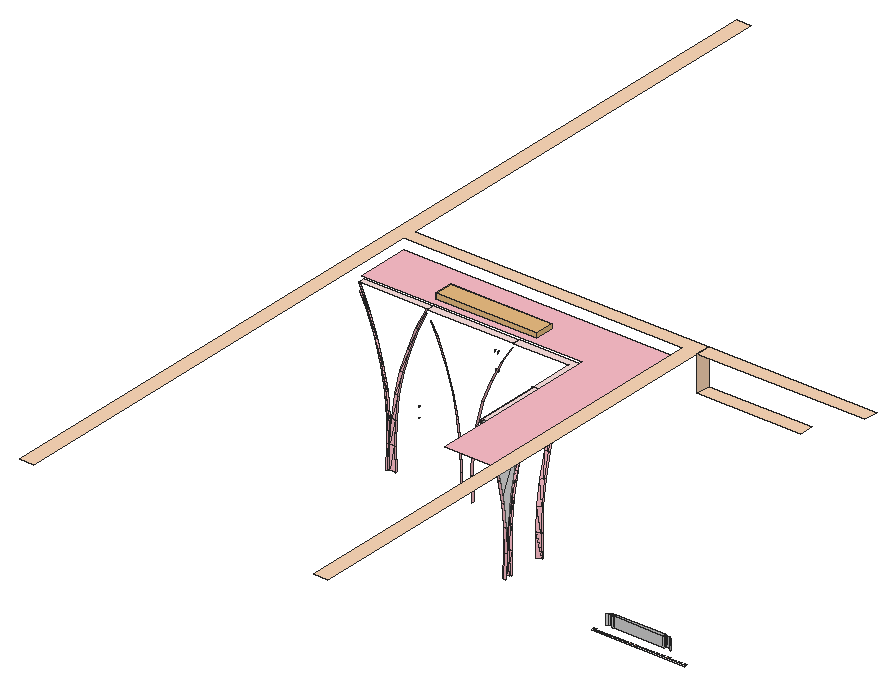
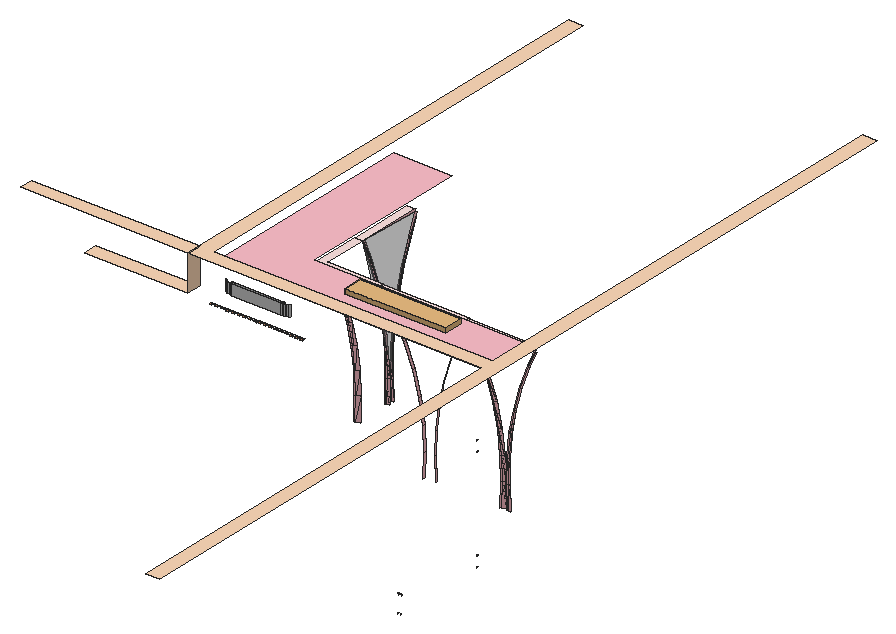
# SketchUp Ruby script. Lengths in inches.
U = 1.inch
M = Sketchup.active_model
def pt(a) = Geom::Point3d.new(a.map { |v| v * U })
def face(e, loops, mat)
  f = e.add_face(loops[0].map { |a| pt(a) })
  loops[1..].each { |l| e.add_face(l.map { |a| pt(a) }).erase! }
  f.material = f.back_material = mat if mat
  f
end
# faces: each face lists its corners as indices into pts; further lists are holes
def faces(e, pts, list, mat = nil) = list.each { |f| face(e, (f[0].is_a?(Array) ? f : [f]).map { |l| l.map { |i| pts[i] } }, mat) }
# xy, xz, yz: faces in a plane at the given z, y or x. An outline is a flat list of corners, or four numbers for a rectangle; further outlines are holes
def ring(l) = l.size == 4 ? [[l[0], l[1]], [l[2], l[1]], [l[2], l[3]], [l[0], l[3]]] : l.each_slice(2).to_a
def flat(e, list, mat, &to3) = list.each { |f| face(e, (f[0].is_a?(Array) ? f : [f]).map { |l| ring(l).map { |u, v| to3.(u, v) } }, mat) }
def xy(e, z, list, mat = nil) = flat(e, list, mat) { |x, y| [x, y, z] }
def xz(e, y, list, mat = nil) = flat(e, list, mat) { |x, z| [x, y, z] }
def yz(e, x, list, mat = nil) = flat(e, list, mat) { |y, z| [x, y, z] }
def lines(e, pts, list) = list.each { |a, b| e.add_line(pt(pts[a]), pt(pts[b])) }
# prism: a flat outline (further loops are holes) pulled along v
def prism(e, loops, v, mat = nil)
  f = face(e, loops, mat); d = Geom::Vector3d.new(v.map { |x| x * U })
  f.pushpull(f.normal.samedirection?(d) ? d.length : -d.length)
end
def box(e, o, s, mat = nil) = prism(e, [[o, [o[0] + s[0], o[1], o[2]], [o[0] + s[0], o[1] + s[1], o[2]], [o[0], o[1] + s[1], o[2]]]], [0, 0, s[2]], mat)
def at(x, y, z, deg = 0) = Geom::Transformation.translation(pt([x, y, z])) * Geom::Transformation.rotation(ORIGIN, Z_AXIS, deg.degrees)
def axes(o, x, y, z) = Geom::Transformation.new([*x, 0, *y, 0, *z, 0, *pt(o).to_a, 1])
def part(name) = M.definitions.add(name)
# library, detail: a bought-in or finely detailed component or shape, given as its bounding box
def library(name, o, s) = part(name).tap { |d| box(d.entities, o, s) }
def detail(e, o, s) = box(e.add_group.entities, o, s)
def put(e, d, t, mat = nil) = e.add_instance(d, t).tap { |i| i.material = mat if mat }
def group(e, t, mat = nil) = e.add_group.tap { |g| g.transformation = t; g.material = mat if mat }.entities
root = M.entities
M.materials.add("Material \#1").color = [140, 140, 140]
M.materials.add("[0006_Pink]").color = [255, 192, 203]
M.materials.add("[0007_MistyRose]").color = [255, 228, 225]
M.materials.add("[0010_Snow]").color = [255, 250, 250]
M.materials.add("[0027_PeachPuff]").color = [255, 218, 185]
M.materials.add("[Carrera Marble]").color = [207, 207, 207]
M.materials.add("[Translucent Glass Gray]").color = [128, 128, 128]
M.materials["[Translucent Glass Gray]"].alpha = 0.5
M.materials.add("[Wood Veneer 02]").color = [190, 128, 91]
c1 = library("wardrobe",[0.19,0,0],[43.3,8.22,2])
xy(root,47.11,[[363.16,355.99,363.12,356,363.12,356.03],[363.16,355.99,363.12,356.03,363.16,356.01],[363.16,355.99,363.16,356.01,363.2,356],[363.12,356,363.08,356.05,363.09,356.07],[363.12,356,363.09,356.07,363.12,356.03],
  [363.2,356,363.16,356.01,363.19,356.03],[363.2,356,363.19,356.03,363.23,356.05],[363.19,356.03,363.22,356.07,363.23,356.05],[363.08,356.05,363.06,356.12,363.07,356.13],[363.08,356.05,363.07,356.13,363.09,356.07],
  [363.23,356.05,363.22,356.07,363.26,356.12],[363.22,356.07,363.25,356.13,363.26,356.12],[363.06,356.12,363.04,356.2,363.06,356.2],[363.06,356.12,363.06,356.2,363.07,356.13],[363.26,356.12,363.25,356.13,363.27,356.2],
  [363.25,356.13,363.26,356.2,363.27,356.2],[363.04,356.2,363.04,356.29,363.06,356.28],[363.04,356.2,363.06,356.28,363.06,356.2],[363.26,356.2,363.26,356.28,363.27,356.29],[363.26,356.2,363.27,356.29,363.27,356.2],
  [363.06,356.28,363.04,356.29,363.07,356.36],[363.26,356.28,363.25,356.36,363.26,356.37],[363.26,356.28,363.26,356.37,363.27,356.29],[363.04,356.29,363.06,356.37,363.07,356.36],[363.07,356.36,363.06,356.37,363.09,356.42],
  [363.25,356.36,363.22,356.42,363.23,356.4375],[363.25,356.36,363.23,356.4375,363.26,356.37],[363.06,356.37,363.08,356.4375,363.09,356.42],[363.09,356.42,363.08,356.4375,363.12,356.46],[363.22,356.42,363.19,356.46,363.2,356.48],
  [363.22,356.42,363.2,356.48,363.23,356.4375],[363.08,356.4375,363.12,356.48,363.12,356.46],[363.12,356.46,363.12,356.48,363.16,356.47],[363.19,356.46,363.16,356.47,363.16,356.49],[363.19,356.46,363.16,356.49,363.2,356.48],
  [363.16,356.47,363.12,356.48,363.16,356.49]],"Material \#1")
xy(root,47.125,[[363.16,355.99,363.16,356.01,363.12,356],[363.16,355.99,363.19,356.03,363.16,356.01],[363.16,355.99,363.2,356,363.19,356.03],[363.12,356,363.12,356.03,363.08,356.05],[363.12,356,363.16,356.01,363.12,356.03],
  [363.2,356,363.22,356.07,363.19,356.03],[363.2,356,363.23,356.05,363.22,356.07],[363.12,356.03,363.09,356.07,363.08,356.05],[363.08,356.05,363.09,356.07,363.06,356.12],[363.23,356.05,363.25,356.13,363.22,356.07],
  [363.23,356.05,363.26,356.12,363.25,356.13],[363.09,356.07,363.07,356.13,363.06,356.12],[363.06,356.12,363.07,356.13,363.04,356.2],[363.26,356.12,363.26,356.2,363.25,356.13],[363.26,356.12,363.27,356.2,363.26,356.2],
  [363.07,356.13,363.06,356.2,363.04,356.2],[363.04,356.2,363.06,356.2,363.04,356.29],[363.06,356.2,363.06,356.28,363.04,356.29],[363.26,356.2,363.27,356.2,363.26,356.28],[363.27,356.2,363.27,356.29,363.26,356.28],
  [363.06,356.28,363.06,356.37,363.04,356.29],[363.06,356.28,363.07,356.36,363.06,356.37],[363.26,356.28,363.27,356.29,363.25,356.36],[363.27,356.29,363.26,356.37,363.25,356.36],[363.07,356.36,363.08,356.4375,363.06,356.37],
  [363.07,356.36,363.09,356.42,363.08,356.4375],[363.25,356.36,363.26,356.37,363.22,356.42],[363.26,356.37,363.23,356.4375,363.22,356.42],[363.09,356.42,363.12,356.48,363.08,356.4375],[363.09,356.42,363.12,356.46,363.12,356.48],
  [363.22,356.42,363.23,356.4375,363.19,356.46],[363.23,356.4375,363.2,356.48,363.19,356.46],[363.12,356.46,363.16,356.47,363.16,356.49],[363.12,356.46,363.16,356.49,363.12,356.48],[363.19,356.46,363.2,356.48,363.16,356.47],
  [363.16,356.47,363.2,356.48,363.16,356.49]],"Material \#1")
xy(root,50.26,[[502.06,274.78,521.41,275.36],[521.88,274.78,542,275.36]],"[0010_Snow]")
xy(root,50.26,[[502.06,275.36,503.17,276.11],[504.3,275.36,505.41,276.11],[506.54,275.36,507.65,276.11],[508.78,275.36,509.89,276.11],[511.02,275.36,512.13,276.11],
  [513.26,275.36,514.37,276.11],[515.5,275.36,516.61,276.11],[517.74,275.36,518.85,276.11],[519.98,275.36,521.09,276.11],[521.88,275.36,522.99,276.11],
  [524.26,275.36,525.37,276.11],[526.63,275.36,527.74,276.11],[529.01,275.36,530.12,276.11],[531.38,275.36,532.5,276.11],[533.76,275.36,534.87,276.11],
  [536.13,275.36,537.25,276.11],[538.51,275.36,539.62,276.11],[540.89,275.36,542,276.11]],"[Wood Veneer 02]")
xy(root,51.55,[[363.16,355.99,363.12,356,363.16,356.01],[363.16,355.99,363.16,356.01,363.19,356.03],[363.16,355.99,363.19,356.03,363.2,356],[363.12,356,363.08,356.05,363.12,356.03],[363.12,356,363.12,356.03,363.16,356.01],
  [363.2,356,363.19,356.03,363.22,356.07],[363.2,356,363.22,356.07,363.23,356.05],[363.12,356.03,363.08,356.05,363.09,356.07],[363.08,356.05,363.06,356.12,363.09,356.07],[363.23,356.05,363.22,356.07,363.25,356.13],
  [363.23,356.05,363.25,356.13,363.26,356.12],[363.09,356.07,363.06,356.12,363.07,356.13],[363.06,356.12,363.04,356.2,363.07,356.13],[363.26,356.12,363.25,356.13,363.26,356.2],[363.26,356.12,363.26,356.2,363.27,356.2],
  [363.07,356.13,363.04,356.2,363.06,356.2],[363.04,356.2,363.04,356.29,363.06,356.2],[363.06,356.2,363.04,356.29,363.06,356.28],[363.26,356.2,363.26,356.28,363.27,356.2],[363.27,356.2,363.26,356.28,363.27,356.29],
  [363.06,356.28,363.04,356.29,363.06,356.37],[363.06,356.28,363.06,356.37,363.07,356.36],[363.26,356.28,363.25,356.36,363.27,356.29],[363.27,356.29,363.25,356.36,363.26,356.37],[363.07,356.36,363.06,356.37,363.08,356.4375],
  [363.07,356.36,363.08,356.4375,363.09,356.42],[363.25,356.36,363.22,356.42,363.26,356.37],[363.26,356.37,363.22,356.42,363.23,356.4375],[363.09,356.42,363.08,356.4375,363.12,356.48],[363.09,356.42,363.12,356.48,363.12,356.46],
  [363.22,356.42,363.19,356.46,363.23,356.4375],[363.23,356.4375,363.19,356.46,363.2,356.48],[363.12,356.46,363.12,356.48,363.16,356.49],[363.12,356.46,363.16,356.49,363.16,356.47],[363.19,356.46,363.16,356.47,363.2,356.48],
  [363.16,356.47,363.16,356.49,363.2,356.48]],"Material \#1")
xy(root,51.57,[[363.16,355.99,363.12,356.03,363.12,356],[363.16,355.99,363.16,356.01,363.12,356.03],[363.16,355.99,363.2,356,363.16,356.01],[363.12,356,363.09,356.07,363.08,356.05],[363.12,356,363.12,356.03,363.09,356.07],
  [363.2,356,363.19,356.03,363.16,356.01],[363.2,356,363.23,356.05,363.19,356.03],[363.19,356.03,363.23,356.05,363.22,356.07],[363.08,356.05,363.07,356.13,363.06,356.12],[363.08,356.05,363.09,356.07,363.07,356.13],
  [363.23,356.05,363.26,356.12,363.22,356.07],[363.22,356.07,363.26,356.12,363.25,356.13],[363.06,356.12,363.06,356.2,363.04,356.2],[363.06,356.12,363.07,356.13,363.06,356.2],[363.26,356.12,363.27,356.2,363.25,356.13],
  [363.25,356.13,363.27,356.2,363.26,356.2],[363.04,356.2,363.06,356.2,363.06,356.28],[363.04,356.2,363.06,356.28,363.04,356.29],[363.26,356.2,363.27,356.2,363.27,356.29],[363.26,356.2,363.27,356.29,363.26,356.28],
  [363.06,356.28,363.07,356.36,363.04,356.29],[363.26,356.28,363.26,356.37,363.25,356.36],[363.26,356.28,363.27,356.29,363.26,356.37],[363.04,356.29,363.07,356.36,363.06,356.37],[363.07,356.36,363.09,356.42,363.06,356.37],
  [363.25,356.36,363.23,356.4375,363.22,356.42],[363.25,356.36,363.26,356.37,363.23,356.4375],[363.06,356.37,363.09,356.42,363.08,356.4375],[363.09,356.42,363.12,356.46,363.08,356.4375],[363.22,356.42,363.2,356.48,363.19,356.46],
  [363.22,356.42,363.23,356.4375,363.2,356.48],[363.08,356.4375,363.12,356.46,363.12,356.48],[363.12,356.46,363.16,356.47,363.12,356.48],[363.19,356.46,363.16,356.49,363.16,356.47],[363.19,356.46,363.2,356.48,363.16,356.49],
  [363.16,356.47,363.16,356.49,363.12,356.48]],"Material \#1")
xy(root,91.49,[[363.16,355.99,363.12,356,363.12,356.03],[363.16,355.99,363.12,356.03,363.16,356.01],[363.16,355.99,363.16,356.01,363.2,356],[363.12,356,363.08,356.05,363.09,356.07],[363.12,356,363.09,356.07,363.12,356.03],
  [363.2,356,363.16,356.01,363.19,356.03],[363.2,356,363.19,356.03,363.23,356.05],[363.19,356.03,363.22,356.07,363.23,356.05],[363.08,356.05,363.06,356.12,363.07,356.13],[363.08,356.05,363.07,356.13,363.09,356.07],
  [363.23,356.05,363.22,356.07,363.26,356.12],[363.22,356.07,363.25,356.13,363.26,356.12],[363.06,356.12,363.04,356.2,363.06,356.2],[363.06,356.12,363.06,356.2,363.07,356.13],[363.26,356.12,363.25,356.13,363.27,356.2],
  [363.25,356.13,363.26,356.2,363.27,356.2],[363.04,356.2,363.04,356.29,363.06,356.28],[363.04,356.2,363.06,356.28,363.06,356.2],[363.26,356.2,363.26,356.28,363.27,356.29],[363.26,356.2,363.27,356.29,363.27,356.2],
  [363.06,356.28,363.04,356.29,363.07,356.36],[363.26,356.28,363.25,356.36,363.26,356.37],[363.26,356.28,363.26,356.37,363.27,356.29],[363.04,356.29,363.06,356.37,363.07,356.36],[363.07,356.36,363.06,356.37,363.09,356.42],
  [363.25,356.36,363.22,356.42,363.23,356.4375],[363.25,356.36,363.23,356.4375,363.26,356.37],[363.06,356.37,363.08,356.4375,363.09,356.42],[363.09,356.42,363.08,356.4375,363.12,356.46],[363.22,356.42,363.19,356.46,363.2,356.48],
  [363.22,356.42,363.2,356.48,363.23,356.4375],[363.08,356.4375,363.12,356.48,363.12,356.46],[363.12,356.46,363.12,356.48,363.16,356.47],[363.19,356.46,363.16,356.47,363.16,356.49],[363.19,356.46,363.16,356.49,363.2,356.48],
  [363.16,356.47,363.12,356.48,363.16,356.49]],"Material \#1")
xy(root,91.51,[[363.16,355.99,363.16,356.01,363.12,356],[363.16,355.99,363.19,356.03,363.16,356.01],[363.16,355.99,363.2,356,363.19,356.03],[363.12,356,363.12,356.03,363.08,356.05],[363.12,356,363.16,356.01,363.12,356.03],
  [363.2,356,363.22,356.07,363.19,356.03],[363.2,356,363.23,356.05,363.22,356.07],[363.12,356.03,363.09,356.07,363.08,356.05],[363.08,356.05,363.09,356.07,363.06,356.12],[363.23,356.05,363.25,356.13,363.22,356.07],
  [363.23,356.05,363.26,356.12,363.25,356.13],[363.09,356.07,363.07,356.13,363.06,356.12],[363.06,356.12,363.07,356.13,363.04,356.2],[363.26,356.12,363.26,356.2,363.25,356.13],[363.26,356.12,363.27,356.2,363.26,356.2],
  [363.07,356.13,363.06,356.2,363.04,356.2],[363.04,356.2,363.06,356.2,363.04,356.29],[363.06,356.2,363.06,356.28,363.04,356.29],[363.26,356.2,363.27,356.2,363.26,356.28],[363.27,356.2,363.27,356.29,363.26,356.28],
  [363.06,356.28,363.06,356.37,363.04,356.29],[363.06,356.28,363.07,356.36,363.06,356.37],[363.26,356.28,363.27,356.29,363.25,356.36],[363.27,356.29,363.26,356.37,363.25,356.36],[363.07,356.36,363.08,356.4375,363.06,356.37],
  [363.07,356.36,363.09,356.42,363.08,356.4375],[363.25,356.36,363.26,356.37,363.22,356.42],[363.26,356.37,363.23,356.4375,363.22,356.42],[363.09,356.42,363.12,356.48,363.08,356.4375],[363.09,356.42,363.12,356.46,363.12,356.48],
  [363.22,356.42,363.23,356.4375,363.19,356.46],[363.23,356.4375,363.2,356.48,363.19,356.46],[363.12,356.46,363.16,356.47,363.16,356.49],[363.12,356.46,363.16,356.49,363.12,356.48],[363.19,356.46,363.2,356.48,363.16,356.47],
  [363.16,356.47,363.2,356.48,363.16,356.49]],"Material \#1")
xy(root,95.93,[[363.16,355.99,363.12,356,363.16,356.01],[363.16,355.99,363.16,356.01,363.19,356.03],[363.16,355.99,363.19,356.03,363.2,356],[363.12,356,363.08,356.05,363.12,356.03],[363.12,356,363.12,356.03,363.16,356.01],
  [363.2,356,363.19,356.03,363.22,356.07],[363.2,356,363.22,356.07,363.23,356.05],[363.12,356.03,363.08,356.05,363.09,356.07],[363.08,356.05,363.06,356.12,363.09,356.07],[363.23,356.05,363.22,356.07,363.25,356.13],
  [363.23,356.05,363.25,356.13,363.26,356.12],[363.09,356.07,363.06,356.12,363.07,356.13],[363.06,356.12,363.04,356.2,363.07,356.13],[363.26,356.12,363.25,356.13,363.26,356.2],[363.26,356.12,363.26,356.2,363.27,356.2],
  [363.07,356.13,363.04,356.2,363.06,356.2],[363.04,356.2,363.04,356.29,363.06,356.2],[363.06,356.2,363.04,356.29,363.06,356.28],[363.26,356.2,363.26,356.28,363.27,356.2],[363.27,356.2,363.26,356.28,363.27,356.29],
  [363.06,356.28,363.04,356.29,363.06,356.37],[363.06,356.28,363.06,356.37,363.07,356.36],[363.26,356.28,363.25,356.36,363.27,356.29],[363.27,356.29,363.25,356.36,363.26,356.37],[363.07,356.36,363.06,356.37,363.08,356.4375],
  [363.07,356.36,363.08,356.4375,363.09,356.42],[363.25,356.36,363.22,356.42,363.26,356.37],[363.26,356.37,363.22,356.42,363.23,356.4375],[363.09,356.42,363.08,356.4375,363.12,356.48],[363.09,356.42,363.12,356.48,363.12,356.46],
  [363.22,356.42,363.19,356.46,363.23,356.4375],[363.23,356.4375,363.19,356.46,363.2,356.48],[363.12,356.46,363.12,356.48,363.16,356.49],[363.12,356.46,363.16,356.49,363.16,356.47],[363.19,356.46,363.16,356.47,363.2,356.48],
  [363.16,356.47,363.16,356.49,363.2,356.48]],"Material \#1")
xy(root,95.95,[[363.16,355.99,363.12,356.03,363.12,356],[363.16,355.99,363.16,356.01,363.12,356.03],[363.16,355.99,363.2,356,363.16,356.01],[363.12,356,363.09,356.07,363.08,356.05],[363.12,356,363.12,356.03,363.09,356.07],
  [363.2,356,363.19,356.03,363.16,356.01],[363.2,356,363.23,356.05,363.19,356.03],[363.19,356.03,363.23,356.05,363.22,356.07],[363.08,356.05,363.07,356.13,363.06,356.12],[363.08,356.05,363.09,356.07,363.07,356.13],
  [363.23,356.05,363.26,356.12,363.22,356.07],[363.22,356.07,363.26,356.12,363.25,356.13],[363.06,356.12,363.06,356.2,363.04,356.2],[363.06,356.12,363.07,356.13,363.06,356.2],[363.26,356.12,363.27,356.2,363.25,356.13],
  [363.25,356.13,363.27,356.2,363.26,356.2],[363.04,356.2,363.06,356.2,363.06,356.28],[363.04,356.2,363.06,356.28,363.04,356.29],[363.26,356.2,363.27,356.2,363.27,356.29],[363.26,356.2,363.27,356.29,363.26,356.28],
  [363.06,356.28,363.07,356.36,363.04,356.29],[363.26,356.28,363.26,356.37,363.25,356.36],[363.26,356.28,363.27,356.29,363.26,356.37],[363.04,356.29,363.07,356.36,363.06,356.37],[363.07,356.36,363.09,356.42,363.06,356.37],
  [363.25,356.36,363.23,356.4375,363.22,356.42],[363.25,356.36,363.26,356.37,363.23,356.4375],[363.06,356.37,363.09,356.42,363.08,356.4375],[363.09,356.42,363.12,356.46,363.08,356.4375],[363.22,356.42,363.2,356.48,363.19,356.46],
  [363.22,356.42,363.23,356.4375,363.2,356.48],[363.08,356.4375,363.12,356.46,363.12,356.48],[363.12,356.46,363.16,356.47,363.12,356.48],[363.19,356.46,363.16,356.49,363.16,356.47],[363.19,356.46,363.2,356.48,363.16,356.49],
  [363.16,356.47,363.16,356.49,363.12,356.48]],"Material \#1")
xy(root,105.875,[[490.5625,345.9375,534.83,351.9375]],"[0027_PeachPuff]")
xy(root,115.8125,[[456.0625,273.46,459.4375,301.21],[456,301.65,459.4375,301.65,459.4375,323.46,432.3125,323.46,432.3125,320.15,456,320.15],[395.4375,320.52,431.8125,323.46],[365.5625,321.02,394.9375,323.46]],"[0007_MistyRose]")
xy(root,116.8125,[[459.4375,249.21,484.5625,249.21,484.5625,345.9375,364.5625,345.9375,364.5625,323.46,459.4375,323.46]],"[0006_Pink]")
xy(root,121.1875,[[358.5625,147.9375,364.5625,147.9375,364.5625,345.9375,484.5625,345.9375,484.5625,147.9375,490.5625,147.9375,490.5625,351.9375,364.5625,351.9375,364.5625,531.9375,358.5625,531.9375],[490.5625,345.9375,562.5625,351.9375]],"[0027_PeachPuff]")
xz(root,273.13,[[512.86,55.54,533.78,59.98]],"[Carrera Marble]")
xz(root,274.24,[[512.86,55.54,533.78,59.98]],"[Carrera Marble]")
yz(root,362.7,[[397.13,54.24,397.15,54.24,397.16,54.4],[397.13,54.24,397.16,54.4,397.15,54.4],[397.15,54.4,397.16,54.4,397.2,54.54],[397.15,54.4,397.2,54.54,397.1875,54.54],[397.1875,54.54,397.2,54.54,397.27,54.67],
  [397.1875,54.54,397.27,54.67,397.25,54.68],[397.27,54.67,397.35,54.79,397.25,54.68],[397.25,54.68,397.35,54.79,397.34,54.8],[397.35,54.79,397.46,54.89,397.34,54.8],[397.34,54.8,397.46,54.89,397.45,54.9],
  [397.46,54.89,397.58,54.98,397.45,54.9],[397.45,54.9,397.58,54.98,397.57,54.99],[397.58,54.98,397.71,55.04,397.57,54.99],[397.57,54.99,397.71,55.04,397.71,55.05]],"Material \#1")
yz(root,362.9,[[397.74,47.14,397.7,47.21,397.68,47.3],[397.7,47.21,397.68,47.25,397.68,47.3],[397.74,47.21,397.68,47.3,397.72,47.27],[397.72,47.27,397.68,47.3,397.71,47.34],[397.68,47.3,397.67,47.34,397.68,47.42],
  [397.68,47.3,397.68,47.42,397.75,47.55],[397.68,47.3,397.72,47.41,397.71,47.34],[397.68,47.3,397.75,47.55,397.72,47.41],[397.68,47.42,397.71,47.49,397.75,47.55]],"Material \#1")
yz(root,363.82,[[397.74,47.14,397.68,47.3,397.7,47.21],[397.7,47.21,397.68,47.3,397.68,47.25],[397.74,47.21,397.72,47.27,397.68,47.3],[397.72,47.27,397.71,47.34,397.68,47.3],[397.68,47.3,397.68,47.42,397.67,47.34],
  [397.68,47.3,397.71,47.34,397.72,47.41],[397.68,47.3,397.72,47.41,397.75,47.55],[397.68,47.3,397.75,47.55,397.68,47.42],[397.68,47.42,397.75,47.55,397.71,47.49]],"Material \#1")
yz(root,364.03,[[397.13,54.24,397.15,54.4,397.16,54.4],[397.13,54.24,397.16,54.4,397.15,54.24],[397.15,54.4,397.1875,54.54,397.2,54.54],[397.15,54.4,397.2,54.54,397.16,54.4],[397.1875,54.54,397.25,54.68,397.27,54.67],
  [397.1875,54.54,397.27,54.67,397.2,54.54],[397.27,54.67,397.25,54.68,397.35,54.79],[397.25,54.68,397.34,54.8,397.35,54.79],[397.35,54.79,397.34,54.8,397.46,54.89],[397.34,54.8,397.45,54.9,397.46,54.89],
  [397.46,54.89,397.45,54.9,397.58,54.98],[397.45,54.9,397.57,54.99,397.58,54.98],[397.58,54.98,397.57,54.99,397.71,55.04],[397.57,54.99,397.71,55.05,397.71,55.04]],"Material \#1")
yz(root,364.05,[[397.74,47.14,397.7,47.21,397.68,47.3],[397.74,47.14,397.72,47.18,397.7,47.21],[397.7,47.21,397.68,47.25,397.68,47.3],[397.74,47.21,397.68,47.3,397.72,47.27],[397.72,47.27,397.68,47.3,397.71,47.34],
  [397.68,47.3,397.67,47.34,397.68,47.42],[397.68,47.3,397.68,47.42,397.75,47.55],[397.68,47.3,397.72,47.41,397.71,47.34],[397.68,47.3,397.74,47.47,397.72,47.41],[397.68,47.3,397.75,47.55,397.74,47.47],
  [397.68,47.42,397.71,47.49,397.75,47.55]],"Material \#1")
yz(root,456,[[316.19,106.54,320.15,115.8125,319.25,112.22]],"[0006_Pink]")
yz(root,456.0625,[[273.46,114.75,273.46,115.8125,301.21,115.8125]],"[0006_Pink]")
yz(root,490.5625,[[345.9375,105.875,351.9375,121.1875]],"[0027_PeachPuff]")
p = [[377.1,320.52,47.87],[378.8,321.02,48.2],[377.74,320.52,57.8125],[413.54,320.52,58.16],[414.09,320.52,47.97],[414.09,321.71,47.97],
  [413.54,321.71,58.16],[454.3,304.72,48.08],[454.55,304.27,58.16],[456,305.625,48.16],[455.3125,286.86,48.24],[455.3125,287.21,58.22],
  [454.375,286.86,48.24],[454.63,287.21,58.22],[456,305.18,58.16],[456.75,305.18,58.16],[456.75,305.625,48.16],[379.1875,321.02,58.16],
  [380.91,321.02,48.16],[379.21,320.52,48.51],[380.5,321.02,58.16],[381.39,321.02,48.2],[380.98,321.02,58.16],[380.98,320.52,58.16],
  [381.39,320.52,48.2],[409.22,320.52,48.2],[409.65,320.52,58.16],[409.65,320.9,58.16],[409.22,320.9,48.2],[456.0625,286.46,48.27],
  [456.0625,286.81,58.22],[455.3125,286.81,58.22],[455.3125,286.46,48.27],[454.31,289.38,48.27],[454.55,289.04,58.16],[455.3125,289.39,48.27],
  [456,289.58,58.16],[455.3125,289.05,58.16],[456,289.92,48.31],[455.32,289.92,48.31],[455.32,289.58,58.16],[378.52,321.02,58.16],
  [378.14,321.02,48.25],[378.14,320.52,48.25],[378.52,320.52,58.16],[379.05,320.52,58.52],[537.6,272.9375,55.54],[537.07,273.32,55.54],
  [537.07,273.32,59.98],[537.6,272.9375,59.98],[512.04,273.04,55.54],[512.45,273.11,55.54],[512.45,273.11,59.98],[512.04,273.04,59.98],
  [534.3125,273.1,55.54],[534.83,273.02,55.54],[534.83,273.02,59.98],[534.3125,273.1,59.98],[510.1,273.47,55.54],[509.65,273.15,55.54],
  [509.65,273.15,59.98],[510.1,273.47,59.98],[512.86,273.13,55.54],[512.86,273.13,59.98],[533.78,273.13,55.54],[533.78,273.13,59.98],
  [536.48,273.64,55.54],[536.48,273.64,59.98],[510.59,273.74,55.54],[510.59,273.74,59.98],[535.85,273.9,55.54],[535.85,273.9,59.98],
  [511.125,273.95,55.54],[511.125,273.95,59.98],[535.18,274.09,55.54],[535.18,274.09,59.98],[511.6875,274.11,55.54],[511.6875,274.11,59.98],
  [512.27,274.21,55.54],[512.27,274.21,59.98],[534.49,274.2,55.54],[534.49,274.2,59.98],[512.86,274.24,55.54],[512.86,274.24,59.98],
  [533.78,274.24,55.54],[533.78,274.24,59.98],[377.6,320.52,67.78],[455.13,285.55,78.09],[456.0625,301.21,115.8125],[454.88,286.78,68.1875],
  [456.0625,286.37,68.15],[455.3125,286.37,68.15],[455.3125,286.77,68.1875],[454.8,289.38,68.04],[456,289.92,68],[455.3125,289.39,68.04],
  [455.32,289.92,68],[454.81,304.72,68.23],[456,305.625,68.15],[456.75,305.625,68.15],[378.8,321.02,68.11],[378.14,321.02,68.06],
  [378.14,320.52,68.06],[380.91,321.02,68.15],[381.39,321.02,68.11],[381.39,320.52,68.11],[409.22,320.52,68.11],[409.22,320.9,68.11],
  [414.09,320.52,68.35],[414.09,321.71,68.35],[379.71,320.52,68.5],[376.7,320.52,77.7],[455.05,290.41,77.88],[456.01,290.94,77.8],
  [455.32,290.42,77.88],[455.32,290.95,77.8],[455.06,306.07,78.22],[456,306.96,78.0625],[456.75,306.96,78.0625],[377.65,321.02,78],
  [376.99,321.02,77.9],[376.99,320.52,77.9],[382.61,321.02,78],[382.61,320.52,78],[407.94,320.52,77.99],[407.94,320.9,77.99],
  [456.0625,285.15,78.03],[455.3125,285.15,78.03],[455.3125,285.54,78.09],[382.13,321.02,78.08],[415.71,320.52,78.42],[415.71,321.71,78.42],
  [381.1875,320.52,78.4],[375.03,320.52,87.52],[456.02,292.64,87.51],[455.33,292.65,87.51],[455.31,292.12,87.62],[455.33,292.12,87.62],
  [375.08,321.02,87.625],[375.08,320.52,87.625],[456.0625,283.14,87.77],[455.3125,283.14,87.77],[375.73,321.02,87.78],[384.63,321.02,87.76],
  [384.63,320.52,87.76],[407.79,320.52,78.69],[405.82,320.52,87.72],[405.82,320.9,87.72],[456.0625,273.46,114.75],[455.38,283.53,87.87],
  [455.625,280.75,97.45],[455.86,277.22,106.79],[455.3125,283.53,87.87],[455.3,308.31,88.06],[456,309.18,87.82],[456.75,309.18,87.82],
  [384.16,321.02,87.875],[383.46,320.52,88.14],[418.41,320.52,88.26],[418.41,321.71,88.26],[456.03,295.01,97.07],[455.34,295.01,97.07],
  [372.61,320.52,97.1875],[374.26,320.52,90.58],[455.5625,294.49,97.22],[455.34,294.5,97.22],[372.43,321.02,97.17],[372.43,320.52,97.17],
  [402.875,320.52,97.23],[402.875,320.9,97.23],[456.0625,280.37,97.33],[455.3125,280.37,97.33],[455.54,311.42,97.65],[456,312.27,97.33],
  [456.75,312.27,97.33],[373.07,321.02,97.375],[387.45,321.02,97.31],[387.45,320.52,97.31],[455.3125,280.75,97.45],[386.99,321.02,97.47],
  [386.53,320.52,97.67],[422.13,320.52,97.76],[422.13,321.71,97.76],[456.05,298.03,106.45],[455.36,298.04,106.45],[455.8125,297.53,106.63],
  [455.36,297.53,106.63],[369.05,321.02,106.49],[369.05,320.52,106.49],[369.45,320.52,106.64],[399.12,320.52,106.46],[399.12,320.9,106.46],
  [456.0625,276.85,106.63],[455.3125,276.85,106.63],[455.78,315.38,106.93],[456,320.15,115.8125],[456,316.19,106.54],[456.75,316.19,106.54],
  [391.03,321.02,106.61],[391.03,320.52,106.61],[369.67,321.02,106.74],[455.3125,277.22,106.79],[390.59,321.02,106.8],[390.36,320.52,106.91],
  [426.85,320.52,106.81],[426.85,321.71,106.81],[456.06,300.68,113.05],[455.37,300.68,113.05],[456.75,319.25,112.22],[456,319.25,112.22],
  [366.23,321.02,112.72],[366.23,320.52,112.72],[396.41,320.52,111.77],[396.41,320.9,111.77],[456.0625,273.86,112.97],[455.3125,273.86,112.97],
  [455.375,301.21,115.8125],[365.5625,320.52,115.8125],[394.45,321.02,113.69],[394.45,320.52,113.69],[365.5625,321.02,115.8125],[455.3125,273.46,114.75],
  [394.9375,321.02,115.8125],[430.96,320.52,112.99],[430.96,321.71,112.99],[394.9375,320.52,115.8125],[456.0625,272.96,115.8125]]
faces(root,p,[[0,1,2],[3,4,5,6],[7,8,9],[10,11,12],[13,12,11],[14,9,8],[15,14,9,16],[17,2,1],
  [18,19,20],[21,22,23,24],[25,26,27,28],[29,30,31,32],[33,34,35],[34,33,36],[37,35,34],[38,36,33],
  [36,38,39,40],[41,42,43,44],[45,20,19],[2,17,86],[30,90,91,31],[89,13,92],[11,92,13],[34,93,37],
  [93,34,94],[36,94,34],[95,37,93],[94,36,40,96],[8,97,14],[98,14,97],[99,98,14,15],[100,86,17],
  [101,41,44,102],[20,45,103],[22,104,105,23],[26,106,107,27],[108,3,6,109],[110,103,45],[86,100,111],[93,112,95],
  [94,113,93],[112,93,113],[114,95,112],[113,94,96,115],[97,116,98],[117,98,116],[118,117,98,99],[119,111,100],
  [120,101,102,121],[104,122,123,105],[106,124,125,107],[90,126,127,91],[87,89,128],[92,128,89],[103,110,129],[130,108,109,131],
  [132,129,110],[111,119,133],[113,134,112],[134,113,115,135],[112,136,114],[136,112,134],[137,114,136],[138,120,121,139],
  [126,140,141,127],[142,133,119],[122,143,144,123],[124,145,146,147,125],[149,87,152],[128,152,87],[116,153,117],[154,117,153],
  [155,154,117,118],[129,132,156],[157,156,132],[158,130,131,159],[134,160,136],[160,134,135,161],[133,142,162,163],[136,164,137],
  [165,137,164],[164,136,160],[166,138,139,163,167],[146,168,169,147],[140,170,171,141],[153,172,154],[173,154,172],[174,173,154,155],
  [175,162,142],[143,176,177,144],[150,149,178],[152,178,149],[156,157,179],[180,179,157],[181,158,159,182],[160,183,164],
  [183,160,161,184],[164,185,165],[186,165,185],[185,164,183],[187,166,167,188],[162,175,189],[168,190,191,169],[170,192,193,171],
  [172,194,173],[195,196,173,194],[197,196,173,174],[176,198,199,177],[200,189,175],[151,150,201],[178,201,150],[179,180,202],
  [203,202,180],[204,181,182,205],[183,206,185],[206,183,184,207],[208,209,196,197],[210,187,188,211],[190,212,213,191],[192,214,215,193],
  [185,88,186],[216,186,88],[88,185,206],[189,200,217],[198,218,219,199],[220,217,200],[148,151,221],[201,221,151],
  [202,203,222],[223,204,205,224],[225,222,203]],"[0006_Pink]")
faces(root,p,[[46,47,48,49],[50,51,52,53],[54,55,56,57],[58,59,60,61],[51,62,63,52],[64,54,57,65],[47,66,67,48],[68,58,61,69],
  [66,70,71,67],[72,68,69,73],[70,74,75,71],[76,72,73,77],[78,76,77,79],[74,80,81,75],[82,78,79,83],[80,84,85,81]],"[Carrera Marble]")
faces(root,p,[[87,88,13,89],[148,88,87,149,150,151]],"[Translucent Glass Gray]")
lines(root,p,[[226,148]])
put(root,c1,at(393.55,326.58,116.8125))
